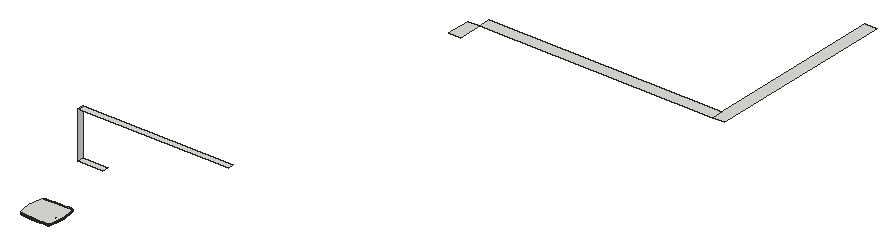
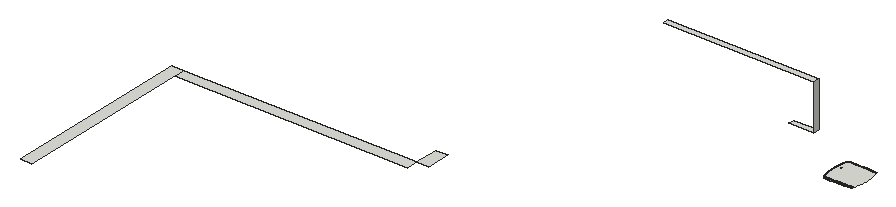
# SketchUp Ruby script. Lengths in inches.
U = 1.inch
M = Sketchup.active_model
def pt(a) = Geom::Point3d.new(a.map { |v| v * U })
def face(e, loops, mat)
  f = e.add_face(loops[0].map { |a| pt(a) })
  loops[1..].each { |l| e.add_face(l.map { |a| pt(a) }).erase! }
  f.material = f.back_material = mat if mat
  f
end
# faces: each face lists its corners as indices into pts; further lists are holes
def faces(e, pts, list, mat = nil) = list.each { |f| face(e, (f[0].is_a?(Array) ? f : [f]).map { |l| l.map { |i| pts[i] } }, mat) }
# xy, xz, yz: faces in a plane at the given z, y or x. An outline is a flat list of corners, or four numbers for a rectangle; further outlines are holes
def ring(l) = l.size == 4 ? [[l[0], l[1]], [l[2], l[1]], [l[2], l[3]], [l[0], l[3]]] : l.each_slice(2).to_a
def flat(e, list, mat, &to3) = list.each { |f| face(e, (f[0].is_a?(Array) ? f : [f]).map { |l| ring(l).map { |u, v| to3.(u, v) } }, mat) }
def xy(e, z, list, mat = nil) = flat(e, list, mat) { |x, y| [x, y, z] }
def xz(e, y, list, mat = nil) = flat(e, list, mat) { |x, z| [x, y, z] }
def yz(e, x, list, mat = nil) = flat(e, list, mat) { |y, z| [x, y, z] }
def lines(e, pts, list) = list.each { |a, b| e.add_line(pt(pts[a]), pt(pts[b])) }
# prism: a flat outline (further loops are holes) pulled along v
def prism(e, loops, v, mat = nil)
  f = face(e, loops, mat); d = Geom::Vector3d.new(v.map { |x| x * U })
  f.pushpull(f.normal.samedirection?(d) ? d.length : -d.length)
end
def box(e, o, s, mat = nil) = prism(e, [[o, [o[0] + s[0], o[1], o[2]], [o[0] + s[0], o[1] + s[1], o[2]], [o[0], o[1] + s[1], o[2]]]], [0, 0, s[2]], mat)
def at(x, y, z, deg = 0) = Geom::Transformation.translation(pt([x, y, z])) * Geom::Transformation.rotation(ORIGIN, Z_AXIS, deg.degrees)
def axes(o, x, y, z) = Geom::Transformation.new([*x, 0, *y, 0, *z, 0, *pt(o).to_a, 1])
def part(name) = M.definitions.add(name)
# library, detail: a bought-in or finely detailed component or shape, given as its bounding box
def library(name, o, s) = part(name).tap { |d| box(d.entities, o, s) }
def detail(e, o, s) = box(e.add_group.entities, o, s)
def put(e, d, t, mat = nil) = e.add_instance(d, t).tap { |i| i.material = mat if mat }
def group(e, t, mat = nil) = e.add_group.tap { |g| g.transformation = t; g.material = mat if mat }.entities
root = M.entities
xy(root,38.7,[[[351.193,77.093,351.37,77.103,351.53,77.131,351.686,77.176,351.836,77.24,351.977,77.32,352.109,77.416,352.228,77.526,352.335,77.649,352.426,77.783,352.502,77.927,352.56,78.079,352.608,78.26,352.823,79.147,353.02,80.038,353.199,80.932,353.359,81.83,353.5,82.731,353.623,83.635,353.726,84.541,353.811,85.449,353.878,86.359,353.925,87.269,353.953,88.181,353.963,89.093,353.953,90.005,353.925,90.916,353.878,91.827,353.811,92.737,353.726,93.645,353.623,94.551,353.5,95.455,353.359,96.356,353.199,97.254,353.02,98.148,352.823,99.038,352.608,99.926,352.56,100.107,352.502,100.259,352.426,100.402,352.335,100.537,352.228,100.66,352.109,100.77,351.977,100.866,351.836,100.946,351.686,101.009,351.53,101.055,351.37,101.083,351.193,101.093,349.441,101.088,347.676,101.074,345.91,101.051,344.144,101.018,342.379,100.976,340.614,100.925,340.613,100.925,338.849,100.865,337.085,100.795,335.321,100.715,333.557,100.627,331.794,100.529,330.048,100.423,329.964,100.412,329.891,100.394,329.82,100.369,329.753,100.336,329.689,100.296,329.63,100.25,329.576,100.198,329.527,100.141,329.486,100.078,329.451,100.012,329.423,99.942,329.4,99.86,329.364,99.687,329.33,99.504,329.3,99.32,329.275,99.135,329.255,98.95,329.239,98.764,329.228,98.578,329.221,98.391,329.218,98.205,329.221,98.018,329.227,97.832,329.245,97.547,328.999,96.771,328.795,96.084,328.605,95.394,328.428,94.699,328.265,94.002,328.115,93.301,327.978,92.598,327.855,91.892,327.745,91.184,327.649,90.474,327.567,89.763,327.502,89.093,327.567,88.423,327.649,87.711,327.745,87.001,327.855,86.293,327.978,85.588,328.115,84.884,328.265,84.184,328.428,83.486,328.605,82.792,328.795,82.101,328.999,81.415,329.245,80.639,329.227,80.354,329.221,80.167,329.218,79.981,329.221,79.794,329.228,79.608,329.239,79.422,329.255,79.236,329.275,79.051,329.3,78.866,329.33,78.682,329.364,78.499,329.4,78.326,329.423,78.244,329.451,78.174,329.486,78.108,329.527,78.045,329.576,77.988,329.63,77.935,329.689,77.889,329.753,77.85,329.82,77.817,329.891,77.792,329.964,77.774,330.048,77.763,331.794,77.657,333.557,77.559,335.321,77.47,337.085,77.391,338.849,77.321,340.614,77.261,342.379,77.209,344.144,77.167,345.91,77.135,347.676,77.111,349.441,77.097],[350.05,90.862,350.3,91.737],[349.737,90.862,349.987,91.737],[350.378,86.33,350.346,86.335,350.316,86.347,350.29,86.367,350.27,86.393,350.258,86.423,350.253,86.455,350.258,86.488,350.27,86.518,350.29,86.544,350.316,86.564,350.346,86.576,350.378,86.58,350.411,86.576,350.441,86.564,350.467,86.544,350.487,86.518,350.499,86.488,350.503,86.455,350.499,86.423,350.487,86.393,350.467,86.367,350.441,86.347,350.411,86.335],[350.377,85.627,350.344,85.632,350.314,85.644,350.288,85.664,350.268,85.69,350.256,85.72,350.252,85.752,350.256,85.785,350.268,85.815,350.288,85.841,350.314,85.861,350.344,85.873,350.377,85.877,350.409,85.873,350.439,85.861,350.465,85.841,350.485,85.815,350.497,85.785,350.502,85.752,350.497,85.72,350.485,85.69,350.465,85.664,350.439,85.644,350.409,85.632]]])
xy(root,72,[[353.416,104.359,373.103,108.859]])
xy(root,108,[[353.416,104.359,471,108.859],[471,319.785,480,338.359],[480,338.359,662.396,347.359],[662.396,338.359,671.44,338.359,671.44,486.825,662.44,486.825,662.44,347.359,662.396,347.359]])
yz(root,353.416,[[104.359,72,108.859,108]])
p = [[345.904,76.767,38.259],[345.903,76.727,38.171],[344.136,76.76,38.171],[344.137,76.799,38.259],[351.81,76.829,38.259],[351.823,76.792,38.171],
  [351.622,76.733,38.171],[351.613,76.772,38.259],[342.369,76.842,38.259],[342.368,76.802,38.171],[340.601,76.853,38.171],[340.602,76.893,38.259],
  [351.998,76.909,38.259],[352.016,76.874,38.171],[338.836,76.954,38.259],[338.834,76.914,38.171],[337.068,76.984,38.171],[337.069,77.024,38.259],
  [352.177,77.01,38.259],[352.198,76.977,38.171],[335.301,77.063,38.171],[335.303,77.103,38.259],[352.342,77.131,38.259],[352.367,77.1,38.171],
  [333.536,77.152,38.171],[333.538,77.192,38.259],[352.493,77.269,38.259],[352.521,77.242,38.171],[331.77,77.25,38.171],[331.773,77.29,38.259],
  [352.627,77.424,38.259],[352.658,77.4,38.171],[352.742,77.594,38.259],[352.776,77.573,38.171],[352.837,77.775,38.259],[352.874,77.758,38.171],
  [352.911,77.966,38.259],[352.949,77.954,38.171],[352.964,78.17,38.259],[353.003,78.16,38.171],[353.182,79.064,38.259],[353.221,79.055,38.171],
  [353.38,79.962,38.259],[353.419,79.954,38.171],[353.56,80.864,38.259],[353.6,80.857,38.171],[353.722,81.769,38.259],[353.761,81.763,38.171],
  [353.864,82.678,38.259],[353.904,82.672,38.171],[353.988,83.589,38.259],[354.027,83.584,38.171],[354.092,84.503,38.259],[354.132,84.499,38.171],
  [354.178,85.418,38.259],[354.218,85.415,38.171],[354.245,86.336,38.259],[354.285,86.333,38.171],[354.292,87.254,38.259],[354.332,87.252,38.171],
  [354.321,88.173,38.259],[354.361,88.172,38.171],[354.331,89.093,38.259],[354.37,89.093,38.171],[354.321,90.012,38.259],[354.361,90.013,38.171],
  [354.292,90.932,38.259],[354.332,90.933,38.171],[354.245,91.85,38.259],[354.285,91.853,38.171],[354.178,92.767,38.259],[354.218,92.771,38.171],
  [354.092,93.683,38.259],[354.132,93.687,38.171],[353.988,94.597,38.259],[354.027,94.602,38.171],[353.864,95.508,38.259],[353.904,95.514,38.171],
  [353.722,96.416,38.259],[353.761,96.423,38.171],[353.56,97.322,38.259],[353.6,97.329,38.171],[353.38,98.224,38.259],[353.419,98.232,38.171],
  [353.182,99.122,38.259],[353.221,99.131,38.171],[352.964,100.016,38.259],[353.003,100.025,38.171],[352.911,100.22,38.259],[352.949,100.232,38.171],
  [352.837,100.411,38.259],[352.874,100.427,38.171],[352.742,100.592,38.259],[352.776,100.613,38.171],[352.627,100.761,38.259],[352.658,100.786,38.171],
  [352.493,100.916,38.259],[352.521,100.944,38.171],[331.773,100.896,38.259],[331.77,100.936,38.171],[333.536,101.034,38.171],[333.538,100.994,38.259],
  [352.342,101.055,38.259],[352.367,101.086,38.171],[335.301,101.123,38.171],[335.303,101.083,38.259],[337.068,101.202,38.171],[337.069,101.162,38.259],
  [352.177,101.176,38.259],[352.198,101.209,38.171],[338.834,101.272,38.171],[338.836,101.232,38.259],[340.601,101.333,38.171],[340.602,101.293,38.259],
  [351.998,101.276,38.259],[352.016,101.312,38.171],[342.368,101.384,38.171],[342.369,101.344,38.259],[344.136,101.426,38.171],[344.137,101.386,38.259],
  [351.81,101.356,38.259],[351.823,101.394,38.171],[345.903,101.459,38.171],[345.904,101.419,38.259],[347.671,101.482,38.171],[347.672,101.442,38.259],
  [349.439,101.496,38.171],[349.439,101.456,38.259],[351.204,101.461,38.259],[351.205,101.501,38.171],[351.416,101.489,38.171],[351.412,101.449,38.259],
  [351.622,101.453,38.171],[351.613,101.414,38.259],[347.672,76.79,38.344],[347.672,76.743,38.259],[345.905,76.813,38.344],[351.603,76.817,38.344],
  [351.412,76.737,38.259],[351.406,76.783,38.344],[342.371,76.888,38.344],[340.604,76.939,38.344],[344.138,76.846,38.344],[344.139,76.899,38.424],
  [342.372,76.941,38.424],[345.906,76.866,38.424],[347.673,76.843,38.424],[349.44,76.829,38.424],[349.44,76.776,38.344],[351.201,76.824,38.424],
  [351.202,76.771,38.344],[351.4,76.836,38.424],[351.591,76.869,38.424],[351.794,76.873,38.344],[351.776,76.923,38.424],[351.978,76.951,38.344],
  [338.837,77,38.344],[340.605,76.992,38.424],[338.839,77.053,38.424],[351.954,76.999,38.424],[352.151,77.049,38.344],[337.071,77.07,38.344],
  [335.305,77.149,38.344],[337.073,77.123,38.424],[352.123,77.094,38.424],[352.279,77.208,38.424],[352.3125,77.167,38.344],[333.54,77.238,38.344],
  [335.308,77.202,38.424],[333.543,77.291,38.424],[352.459,77.302,38.344],[331.775,77.336,38.344],[331.778,77.389,38.424],[352.421,77.339,38.424],
  [330.012,77.397,38.259],[330.017,77.443,38.344],[330.022,77.496,38.424],[352.548,77.485,38.424],[352.59,77.453,38.344],[352.702,77.617,38.344],
  [352.657,77.645,38.424],[352.795,77.794,38.344],[352.747,77.816,38.424],[352.816,77.996,38.424],[352.867,77.98,38.344],[352.868,78.194,38.424],
  [352.919,78.182,38.344],[353.136,79.075,38.344],[353.085,79.087,38.424],[353.335,79.972,38.344],[353.283,79.982,38.424],[353.515,80.873,38.344],
  [353.463,80.882,38.424],[353.676,81.777,38.344],[353.624,81.786,38.424],[353.766,82.692,38.424],[353.818,82.685,38.344],[353.942,83.595,38.344],
  [353.889,83.601,38.424],[354.046,84.508,38.344],[353.994,84.513,38.424],[354.132,85.422,38.344],[354.079,85.427,38.424],[354.198,86.339,38.344],
  [354.146,86.342,38.424],[354.193,87.258,38.424],[354.246,87.256,38.344],[354.275,88.174,38.344],[354.222,88.175,38.424],[354.231,89.093,38.424],
  [354.284,89.093,38.344],[354.222,90.01,38.424],[354.275,90.012,38.344],[354.193,90.928,38.424],[354.246,90.93,38.344],[354.146,91.844,38.424],
  [354.198,91.847,38.344],[354.079,92.759,38.424],[354.132,92.763,38.344],[353.994,93.673,38.424],[354.046,93.678,38.344],[353.889,94.584,38.424],
  [353.942,94.591,38.344],[353.766,95.494,38.424],[353.818,95.501,38.344],[353.624,96.4,38.424],[353.676,96.409,38.344],[353.463,97.303,38.424],
  [353.515,97.313,38.344],[353.283,98.203,38.424],[353.335,98.214,38.344],[353.085,99.099,38.424],[353.136,99.111,38.344],[352.868,99.991,38.424],
  [352.919,100.004,38.344],[352.816,100.189,38.424],[352.867,100.206,38.344],[352.747,100.37,38.424],[352.795,100.392,38.344],[352.657,100.541,38.424],
  [352.702,100.568,38.344],[352.548,100.701,38.424],[352.59,100.733,38.344],[330.022,100.69,38.424],[330.017,100.743,38.344],[331.775,100.85,38.344],
  [331.778,100.797,38.424],[352.421,100.847,38.424],[352.459,100.884,38.344],[333.54,100.948,38.344],[333.543,100.895,38.424],[352.279,100.978,38.424],
  [352.3125,101.019,38.344],[335.305,101.036,38.344],[335.308,100.984,38.424],[337.071,101.116,38.344],[337.073,101.063,38.424],[352.123,101.092,38.424],
  [352.151,101.136,38.344],[338.837,101.186,38.344],[338.839,101.133,38.424],[340.603,101.246,38.344],[340.605,101.194,38.424],[351.954,101.187,38.424],
  [351.978,101.235,38.344],[342.371,101.298,38.344],[342.372,101.245,38.424],[344.138,101.34,38.344],[344.139,101.287,38.424],[351.776,101.263,38.424],
  [351.794,101.3125,38.344],[345.905,101.372,38.344],[345.906,101.32,38.424],[347.672,101.396,38.344],[347.673,101.343,38.424],[349.44,101.41,38.344],
  [349.44,101.357,38.424],[351.4,101.35,38.424],[351.406,101.403,38.344],[351.603,101.369,38.344],[351.591,101.317,38.424],[351.202,101.414,38.344],
  [351.201,101.362,38.424],[347.673,76.902,38.501],[345.907,76.925,38.501],[349.44,76.888,38.501],[351.199,76.883,38.501],[351.393,76.894,38.501],
  [351.577,76.926,38.501],[342.374,77,38.501],[340.607,77.051,38.501],[344.14,76.958,38.501],[351.756,76.979,38.501],[351.928,77.052,38.501],
  [338.841,77.112,38.501],[352.091,77.143,38.501],[337.076,77.182,38.501],[335.311,77.261,38.501],[352.242,77.253,38.501],[333.546,77.35,38.501],
  [352.379,77.38,38.501],[331.782,77.448,38.501],[352.501,77.521,38.501],[330.028,77.554,38.501],[352.606,77.675,38.501],[352.693,77.84,38.501],
  [352.76,78.014,38.501],[352.811,78.209,38.501],[353.028,79.1,38.501],[353.226,79.995,38.501],[353.405,80.893,38.501],[353.566,81.795,38.501],
  [353.708,82.701,38.501],[353.831,83.609,38.501],[353.935,84.519,38.501],[354.02,85.432,38.501],[354.087,86.346,38.501],[354.134,87.261,38.501],
  [354.163,88.177,38.501],[354.172,89.093,38.501],[354.163,90.009,38.501],[354.134,90.925,38.501],[354.087,91.84,38.501],[354.02,92.754,38.501],
  [353.935,93.667,38.501],[353.831,94.577,38.501],[353.708,95.485,38.501],[353.566,96.39,38.501],[353.405,97.292,38.501],[353.226,98.191,38.501],
  [353.028,99.086,38.501],[352.811,99.977,38.501],[352.76,100.171,38.501],[352.693,100.345,38.501],[352.606,100.511,38.501],[352.501,100.665,38.501],
  [330.028,100.631,38.501],[331.782,100.738,38.501],[333.546,100.836,38.501],[352.379,100.806,38.501],[335.311,100.925,38.501],[352.242,100.932,38.501],
  [337.076,101.004,38.501],[352.091,101.042,38.501],[338.841,101.074,38.501],[351.928,101.134,38.501],[340.607,101.135,38.501],[342.374,101.186,38.501],
  [351.756,101.207,38.501],[344.14,101.228,38.501],[345.907,101.261,38.501],[351.577,101.26,38.501],[347.673,101.284,38.501],[349.44,101.298,38.501],
  [351.199,101.303,38.501],[351.393,101.292,38.501],[345.908,76.99,38.573],[344.141,77.022,38.573],[347.674,76.966,38.573],[349.441,76.952,38.573],
  [351.197,76.948,38.573],[351.386,76.959,38.573],[351.5625,76.989,38.573],[351.735,77.04,38.573],[342.375,77.064,38.573],[340.609,77.116,38.573],
  [351.9,77.11,38.573],[338.844,77.176,38.573],[337.079,77.246,38.573],[352.056,77.198,38.573],[352.201,77.303,38.573],[335.314,77.326,38.573],
  [333.549,77.414,38.573],[331.786,77.512,38.573],[352.332,77.425,38.573],[330.034,77.619,38.573],[352.45,77.56,38.573],[352.551,77.709,38.573],
  [352.634,77.867,38.573],[352.699,78.034,38.573],[352.748,78.225,38.573],[352.965,79.115,38.573],[353.162,80.008,38.573],[353.341,80.905,38.573],
  [353.502,81.806,38.573],[353.644,82.71,38.573],[353.767,83.617,38.573],[353.871,84.526,38.573],[353.956,85.437,38.573],[354.022,86.35,38.573],
  [354.07,87.263,38.573],[354.098,88.178,38.573],[354.108,89.093,38.573],[354.098,90.008,38.573],[354.07,90.922,38.573],[354.022,91.836,38.573],
  [353.956,92.749,38.573],[353.871,93.66,38.573],[353.767,94.569,38.573],[353.644,95.476,38.573],[353.502,96.38,38.573],[353.341,97.28,38.573],
  [353.162,98.178,38.573],[352.965,99.071,38.573],[352.748,99.961,38.573],[352.699,100.151,38.573],[352.634,100.319,38.573],[352.551,100.477,38.573],
  [352.45,100.625,38.573],[330.034,100.567,38.573],[331.786,100.674,38.573],[352.332,100.761,38.573],[333.549,100.772,38.573],[335.314,100.86,38.573],
  [352.201,100.882,38.573],[337.079,100.939,38.573],[338.844,101.009,38.573],[352.056,100.988,38.573],[340.608,101.07,38.573],[351.9,101.076,38.573],
  [342.375,101.121,38.573],[344.141,101.163,38.573],[351.5625,101.197,38.573],[351.735,101.146,38.573],[345.908,101.196,38.573],[347.674,101.219,38.573],
  [349.441,101.233,38.573],[351.197,101.238,38.573],[351.386,101.227,38.573],[351.196,77.018,38.639],[349.441,77.022,38.639],[351.378,77.028,38.639],
  [344.143,77.092,38.639],[342.377,77.134,38.639],[345.909,77.06,38.639],[347.675,77.036,38.639],[347.676,77.111,38.7],[345.91,77.135,38.7],
  [349.441,77.097,38.7],[351.193,77.093,38.7],[351.37,77.103,38.7],[351.547,77.057,38.639],[351.53,77.131,38.7],[351.711,77.106,38.639],
  [351.869,77.173,38.639],[340.612,77.186,38.639],[338.846,77.246,38.639],[342.379,77.209,38.7],[340.614,77.261,38.7],[344.144,77.167,38.7],
  [351.686,77.176,38.7],[351.836,77.24,38.7],[352.018,77.257,38.639],[337.082,77.316,38.639],[335.317,77.396,38.639],[338.849,77.321,38.7],
  [337.085,77.391,38.7],[351.977,77.32,38.7],[352.156,77.358,38.639],[333.553,77.484,38.639],[335.321,77.47,38.7],[352.109,77.416,38.7],
  [352.282,77.474,38.639],[331.79,77.582,38.639],[333.557,77.559,38.7],[352.228,77.526,38.7],[352.394,77.603,38.639],[330.041,77.688,38.639],
  [331.794,77.657,38.7],[352.335,77.649,38.7],[330.048,77.763,38.7],[352.426,77.783,38.7],[352.49,77.745,38.639],[352.502,77.927,38.7],
  [352.57,77.896,38.639],[352.56,78.079,38.7],[352.632,78.056,38.639],[352.68,78.242,38.639],[352.608,78.26,38.7],[352.823,79.147,38.7],
  [352.896,79.13,38.639],[353.02,80.038,38.7],[353.094,80.022,38.639],[353.199,80.932,38.7],[353.273,80.918,38.639],[353.359,81.83,38.7],
  [353.433,81.818,38.639],[353.574,82.72,38.639],[353.5,82.731,38.7],[353.623,83.635,38.7],[353.697,83.625,38.639],[353.726,84.541,38.7],
  [353.801,84.533,38.639],[353.811,85.449,38.7],[353.886,85.443,38.639],[353.878,86.359,38.7],[353.952,86.354,38.639],[354,87.266,38.639],
  [353.925,87.269,38.7],[353.953,88.181,38.7],[354.028,88.179,38.639],[354.038,89.093,38.639],[353.963,89.093,38.7],[353.953,90.005,38.7],
  [354.028,90.006,38.639],[353.925,90.916,38.7],[354,90.92,38.639],[353.878,91.827,38.7],[353.952,91.832,38.639],[353.811,92.737,38.7],
  [353.886,92.743,38.639],[353.726,93.645,38.7],[353.801,93.653,38.639],[353.623,94.551,38.7],[353.697,94.56,38.639],[353.5,95.455,38.7],
  [353.574,95.466,38.639],[353.359,96.356,38.7],[353.433,96.368,38.639],[353.199,97.254,38.7],[353.273,97.267,38.639],[353.02,98.148,38.7],
  [353.094,98.163,38.639],[352.823,99.038,38.7],[352.896,99.055,38.639],[352.608,99.926,38.7],[352.68,99.944,38.639],[352.56,100.107,38.7],
  [352.632,100.13,38.639],[352.502,100.259,38.7],[352.57,100.29,38.639],[352.426,100.402,38.7],[352.49,100.441,38.639],[330.048,100.423,38.7],
  [330.041,100.497,38.639],[331.79,100.604,38.639],[331.794,100.529,38.7],[352.335,100.537,38.7],[352.394,100.583,38.639],[333.553,100.702,38.639],
  [333.557,100.627,38.7],[352.228,100.66,38.7],[352.282,100.712,38.639],[335.317,100.79,38.639],[335.321,100.715,38.7],[337.082,100.869,38.639],
  [337.085,100.795,38.7],[352.109,100.77,38.7],[352.156,100.828,38.639],[338.846,100.939,38.639],[338.849,100.865,38.7],[351.977,100.866,38.7],
  [352.018,100.929,38.639],[340.61,101,38.639],[340.613,100.925,38.7],[342.379,100.976,38.7],[340.614,100.925,38.7],[340.612,101,38.639],
  [342.377,101.051,38.639],[351.686,101.009,38.7],[351.711,101.08,38.639],[351.869,101.013,38.639],[351.836,100.946,38.7],[344.143,101.093,38.639],
  [344.144,101.018,38.7],[345.909,101.126,38.639],[345.91,101.051,38.7],[351.53,101.055,38.7],[351.547,101.128,38.639],[347.675,101.149,38.639],
  [347.676,101.074,38.7],[349.441,101.163,38.639],[349.441,101.088,38.7],[351.196,101.168,38.639],[351.193,101.093,38.7],[351.378,101.158,38.639],
  [351.37,101.083,38.7]]
faces(root,p,[[0,1,2,3],[4,5,6,7],[8,9,10,11],[3,2,9,8],[12,13,5,4],[14,15,16,17],[11,10,15,14],[18,19,13,12],
  [17,16,20,21],[22,23,19,18],[21,20,24,25],[26,27,23,22],[25,24,28,29],[30,31,27,26],[32,33,31,30],[34,35,33,32],
  [36,37,35,34],[38,39,37,36],[40,41,39,38],[42,43,41,40],[44,45,43,42],[46,47,45,44],[48,49,47,46],[50,51,49,48],
  [52,53,51,50],[54,55,53,52],[56,57,55,54],[58,59,57,56],[60,61,59,58],[62,63,61,60],[64,65,63,62],[66,67,65,64],
  [68,69,67,66],[70,71,69,68],[72,73,71,70],[74,75,73,72],[76,77,75,74],[78,79,77,76],[80,81,79,78],[82,83,81,80],
  [84,85,83,82],[86,87,85,84],[88,89,87,86],[90,91,89,88],[92,93,91,90],[94,95,93,92],[96,97,95,94],[98,99,100,101],
  [102,103,97,96],[101,100,104,105],[105,104,106,107],[108,109,103,102],[107,106,110,111],[111,110,112,113],[114,115,109,108],[113,112,116,117],
  [117,116,118,119],[120,121,115,114],[119,118,122,123],[123,122,124,125],[125,124,126,127],[128,129,130,131],[131,130,132,133],[133,132,121,120],
  [127,126,129,128],[134,135,0,136],[137,7,138,139],[140,8,11,141],[142,3,8,140],[143,142,140,144],[136,0,3,142],[145,136,142,143],
  [146,134,136,145],[147,148,134,146],[149,150,148,147],[151,139,150,149],[152,137,139,151],[153,4,7,137],[154,153,137,152],[155,12,4,153],
  [141,11,14,156],[157,141,156,158],[144,140,141,157],[159,155,153,154],[160,18,12,155],[161,17,21,162],[156,14,17,161],[158,156,161,163],
  [164,160,155,159],[165,166,160,164],[166,22,18,160],[162,21,25,167],[168,162,167,169],[163,161,162,168],[170,26,22,166],[167,25,29,171],
  [169,167,171,172],[173,170,166,165],[171,29,174,175],[172,171,175,176],[177,178,170,173],[178,30,26,170],[179,32,30,178],[180,179,178,177],
  [181,34,32,179],[182,181,179,180],[183,184,181,182],[184,36,34,181],[185,186,184,183],[186,38,36,184],[187,40,38,186],[188,187,186,185],
  [189,42,40,187],[190,189,187,188],[191,44,42,189],[192,191,189,190],[193,46,44,191],[194,193,191,192],[195,196,193,194],[196,48,46,193],
  [197,50,48,196],[198,197,196,195],[199,52,50,197],[200,199,197,198],[201,54,52,199],[202,201,199,200],[203,56,54,201],[204,203,201,202],
  [205,206,203,204],[206,58,56,203],[207,60,58,206],[208,207,206,205],[209,210,207,208],[210,62,60,207],[211,212,210,209],[212,64,62,210],
  [213,214,212,211],[214,66,64,212],[215,216,214,213],[216,68,66,214],[217,218,216,215],[218,70,68,216],[219,220,218,217],[220,72,70,218],
  [221,222,220,219],[222,74,72,220],[223,224,222,221],[224,76,74,222],[225,226,224,223],[226,78,76,224],[227,228,226,225],[228,80,78,226],
  [229,230,228,227],[230,82,80,228],[231,232,230,229],[232,84,82,230],[233,234,232,231],[234,86,84,232],[235,236,234,233],[236,88,86,234],
  [237,238,236,235],[238,90,88,236],[239,240,238,237],[240,92,90,238],[241,242,240,239],[242,94,92,240],[243,244,245,246],[247,248,242,241],
  [248,96,94,242],[246,245,249,250],[245,98,101,249],[251,252,248,247],[250,249,253,254],[249,101,105,253],[252,102,96,248],[254,253,255,256],
  [253,105,107,255],[257,258,252,251],[258,108,102,252],[256,255,259,260],[255,107,111,259],[260,259,261,262],[263,264,258,257],[264,114,108,258],
  [259,111,113,261],[262,261,265,266],[261,113,117,265],[266,265,267,268],[269,270,264,263],[270,120,114,264],[265,117,119,267],[268,267,271,272],
  [267,119,123,271],[272,271,273,274],[274,273,275,276],[277,278,279,280],[280,279,270,269],[279,133,120,270],[271,123,125,273],[273,125,127,275],
  [276,275,281,282],[275,127,128,281],[282,281,278,277],[281,128,131,278],[278,131,133,279],[283,146,145,284],[285,147,146,283],[286,149,147,285],
  [287,151,149,286],[288,152,151,287],[289,144,157,290],[291,143,144,289],[284,145,143,291],[292,154,152,288],[293,159,154,292],[290,157,158,294],
  [295,164,159,293],[296,163,168,297],[294,158,163,296],[298,165,164,295],[297,168,169,299],[300,173,165,298],[299,169,172,301],[302,177,173,300],
  [301,172,176,303],[304,180,177,302],[305,182,180,304],[306,183,182,305],[307,185,183,306],[308,188,185,307],[309,190,188,308],[310,192,190,309],
  [311,194,192,310],[312,195,194,311],[313,198,195,312],[314,200,198,313],[315,202,200,314],[316,204,202,315],[317,205,204,316],[318,208,205,317],
  [319,209,208,318],[320,211,209,319],[321,213,211,320],[322,215,213,321],[323,217,215,322],[324,219,217,323],[325,221,219,324],[326,223,221,325],
  [327,225,223,326],[328,227,225,327],[329,229,227,328],[330,231,229,329],[331,233,231,330],[332,235,233,331],[333,237,235,332],[334,239,237,333],
  [335,241,239,334],[336,243,246,337],[337,246,250,338],[339,247,241,335],[338,250,254,340],[341,251,247,339],[340,254,256,342],[343,257,251,341],
  [342,256,260,344],[345,263,257,343],[344,260,262,346],[346,262,266,347],[348,269,263,345],[347,266,268,349],[349,268,272,350],[351,280,269,348],
  [350,272,274,352],[352,274,276,353],[353,276,282,354],[354,282,277,355],[355,277,280,351],[356,284,291,357],[358,283,284,356],[359,285,283,358],
  [360,286,285,359],[361,287,286,360],[362,288,287,361],[363,292,288,362],[364,289,290,365],[357,291,289,364],[366,293,292,363],[367,294,296,368],
  [365,290,294,367],[369,295,293,366],[370,298,295,369],[368,296,297,371],[372,299,301,373],[371,297,299,372],[374,300,298,370],[373,301,303,375],
  [376,302,300,374],[377,304,302,376],[378,305,304,377],[379,306,305,378],[380,307,306,379],[381,308,307,380],[382,309,308,381],[383,310,309,382],
  [384,311,310,383],[385,312,311,384],[386,313,312,385],[387,314,313,386],[388,315,314,387],[389,316,315,388],[390,317,316,389],[391,318,317,390],
  [392,319,318,391],[393,320,319,392],[394,321,320,393],[395,322,321,394],[396,323,322,395],[397,324,323,396],[398,325,324,397],[399,326,325,398],
  [400,327,326,399],[401,328,327,400],[402,329,328,401],[403,330,329,402],[404,331,330,403],[405,332,331,404],[406,333,332,405],[407,334,333,406],
  [408,335,334,407],[409,336,337,410],[411,339,335,408],[410,337,338,412],[412,338,340,413],[414,341,339,411],[413,340,342,415],[415,342,344,416],
  [417,343,341,414],[416,344,346,418],[419,345,343,417],[418,346,347,420],[420,347,349,421],[422,351,348,423],[423,348,345,419],[421,349,350,424],
  [424,350,352,425],[425,352,353,426],[426,353,354,427],[427,354,355,428],[428,355,351,422],[429,360,359,430],[431,361,360,429],[432,357,364,433],
  [434,356,357,432],[435,358,356,434],[436,435,434,437],[430,359,358,435],[438,430,435,436],[439,429,430,438],[440,431,429,439],[441,362,361,431],
  [442,441,431,440],[443,363,362,441],[444,366,363,443],[445,365,367,446],[433,364,365,445],[447,433,445,448],[449,432,433,447],[437,434,432,449],
  [450,443,441,442],[451,444,443,450],[452,369,366,444],[453,368,371,454],[446,367,368,453],[455,446,453,456],[448,445,446,455],[457,452,444,451],
  [458,370,369,452],[454,371,372,459],[456,453,454,460],[461,458,452,457],[462,374,370,458],[459,372,373,463],[460,454,459,464],[465,462,458,461],
  [466,376,374,462],[463,373,375,467],[464,459,463,468],[469,466,462,465],[468,463,467,470],[471,472,466,469],[472,377,376,466],[473,474,472,471],
  [474,378,377,472],[475,476,474,473],[476,379,378,474],[477,380,379,476],[478,477,476,475],[479,480,477,478],[480,381,380,477],[481,482,480,479],
  [482,382,381,480],[483,484,482,481],[484,383,382,482],[485,486,484,483],[486,384,383,484],[487,385,384,486],[488,487,486,485],[489,490,487,488],
  [490,386,385,487],[491,492,490,489],[492,387,386,490],[493,494,492,491],[494,388,387,492],[495,496,494,493],[496,389,388,494],[497,390,389,496],
  [498,497,496,495],[499,500,497,498],[500,391,390,497],[501,392,391,500],[502,501,500,499],[503,504,501,502],[504,393,392,501],[505,506,504,503],
  [506,394,393,504],[507,508,506,505],[508,395,394,506],[509,510,508,507],[510,396,395,508],[511,512,510,509],[512,397,396,510],[513,514,512,511],
  [514,398,397,512],[515,516,514,513],[516,399,398,514],[517,518,516,515],[518,400,399,516],[519,520,518,517],[520,401,400,518],[521,522,520,519],
  [522,402,401,520],[523,524,522,521],[524,403,402,522],[525,526,524,523],[526,404,403,524],[527,528,526,525],[528,405,404,526],[529,530,528,527],
  [530,406,405,528],[531,532,530,529],[532,407,406,530],[533,534,535,536],[537,538,532,531],[538,408,407,532],[534,409,410,535],[536,535,539,540],
  [541,542,538,537],[535,410,412,539],[540,539,543,544],[542,411,408,538],[539,412,413,543],[544,543,545,546],[547,548,542,541],[548,414,411,542],
  [543,413,415,545],[546,545,549,550],[551,552,548,547],[552,417,414,548],[545,415,416,549],[549,553,554,550],[416,418,553,549],[555,556,557,558],
  [559,560,561,562],[562,561,552,551],[561,419,417,552],[558,557,418,420],[555,558,563,564],[564,563,565,566],[567,568,560,559],[560,423,419,561],
  [558,420,421,563],[563,421,424,565],[566,565,569,570],[565,424,425,569],[570,569,571,572],[569,425,426,571],[572,571,573,574],[574,573,575,576],
  [576,575,568,567],[575,428,422,568],[568,422,423,560],[571,426,427,573],[573,427,428,575]])
